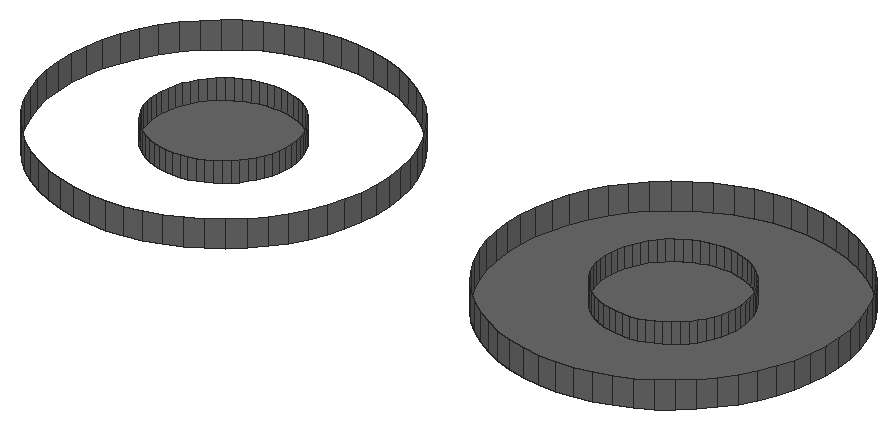
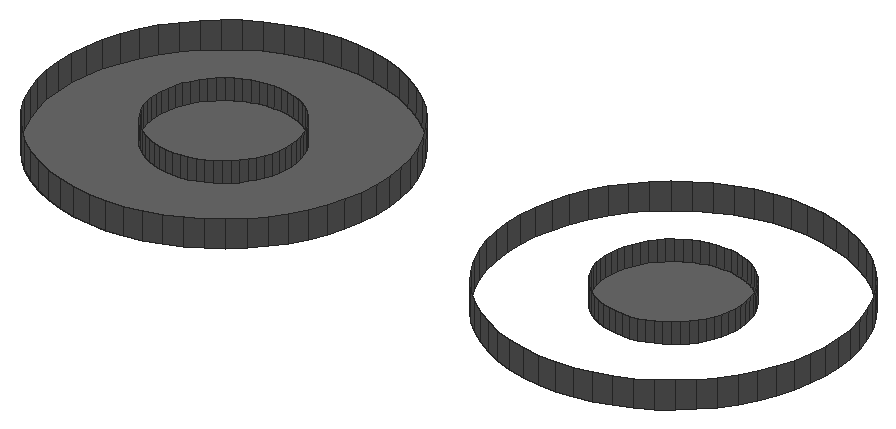
# SketchUp Ruby script. Lengths in inches.
U = 1.inch
M = Sketchup.active_model
def pt(a) = Geom::Point3d.new(a.map { |v| v * U })
def face(e, loops, mat)
  f = e.add_face(loops[0].map { |a| pt(a) })
  loops[1..].each { |l| e.add_face(l.map { |a| pt(a) }).erase! }
  f.material = f.back_material = mat if mat
  f
end
# faces: each face lists its corners as indices into pts; further lists are holes
def faces(e, pts, list, mat = nil) = list.each { |f| face(e, (f[0].is_a?(Array) ? f : [f]).map { |l| l.map { |i| pts[i] } }, mat) }
# xy, xz, yz: faces in a plane at the given z, y or x. An outline is a flat list of corners, or four numbers for a rectangle; further outlines are holes
def ring(l) = l.size == 4 ? [[l[0], l[1]], [l[2], l[1]], [l[2], l[3]], [l[0], l[3]]] : l.each_slice(2).to_a
def flat(e, list, mat, &to3) = list.each { |f| face(e, (f[0].is_a?(Array) ? f : [f]).map { |l| ring(l).map { |u, v| to3.(u, v) } }, mat) }
def xy(e, z, list, mat = nil) = flat(e, list, mat) { |x, y| [x, y, z] }
def xz(e, y, list, mat = nil) = flat(e, list, mat) { |x, z| [x, y, z] }
def yz(e, x, list, mat = nil) = flat(e, list, mat) { |y, z| [x, y, z] }
def lines(e, pts, list) = list.each { |a, b| e.add_line(pt(pts[a]), pt(pts[b])) }
# prism: a flat outline (further loops are holes) pulled along v
def prism(e, loops, v, mat = nil)
  f = face(e, loops, mat); d = Geom::Vector3d.new(v.map { |x| x * U })
  f.pushpull(f.normal.samedirection?(d) ? d.length : -d.length)
end
def box(e, o, s, mat = nil) = prism(e, [[o, [o[0] + s[0], o[1], o[2]], [o[0] + s[0], o[1] + s[1], o[2]], [o[0], o[1] + s[1], o[2]]]], [0, 0, s[2]], mat)
def at(x, y, z, deg = 0) = Geom::Transformation.translation(pt([x, y, z])) * Geom::Transformation.rotation(ORIGIN, Z_AXIS, deg.degrees)
def axes(o, x, y, z) = Geom::Transformation.new([*x, 0, *y, 0, *z, 0, *pt(o).to_a, 1])
def part(name) = M.definitions.add(name)
# library, detail: a bought-in or finely detailed component or shape, given as its bounding box
def library(name, o, s) = part(name).tap { |d| box(d.entities, o, s) }
def detail(e, o, s) = box(e.add_group.entities, o, s)
def put(e, d, t, mat = nil) = e.add_instance(d, t).tap { |i| i.material = mat if mat }
def group(e, t, mat = nil) = e.add_group.tap { |g| g.transformation = t; g.material = mat if mat }.entities
root = M.entities
M.materials.add("[0134_DimGray]").color = [105, 105, 105]
xy(root,118,[[107.89,159.41,106.64,159.53,105.41,159.78,104.21,160.16,103.0625,160.67,101.97,161.29,100.95,162.02,100.01,162.85,99.16,163.78,98.42,164.79,97.78,165.875,97.26,167.02,96.87,168.21,96.6,169.4375,96.46,170.6875,96.45,171.94,96.57,173.19,96.83,174.42,97.21,175.62,97.71,176.77,98.33,177.86,99.0625,178.88,99.9,179.82,100.82,180.67,101.84,181.42,102.92,182.05,104.0625,182.57,105.26,182.97,106.48,183.23,107.73,183.375,108.99,183.38,110.24,183.26,111.47,183.01,112.66,182.625,113.81,182.125,114.91,181.5,115.93,180.77,116.87,179.9375,117.71,179.01,118.46,178,119.09,176.91,119.61,175.77,120.01,174.58,120.28,173.35,120.42,172.1,120.43,170.85,120.3,169.6,120.05,168.37,119.67,167.17,119.17,166.02,118.55,164.93,117.8125,163.91,116.98,162.97,116.05,162.12,115.04,161.375,113.96,160.74,112.8125,160.22,111.62,159.83,110.39,159.56,109.15,159.42]],"[0134_DimGray]")
xy(root,118.5,[[75.77,164.98,76.3,165.02,76.81,165.12,77.31,165.28,77.79,165.48,78.25,165.73,78.68,166.03,79.07,166.38,79.43,166.76,79.75,167.18,80.01,167.625,80.24,168.1,80.41,168.6,80.52,169.11,80.59,169.625,80.6,170.15,80.55,170.67,80.45,171.18,80.3,171.68,80.09,172.17,79.84,172.625,79.54,173.05,79.2,173.45,78.8125,173.8,78.4,174.12,77.95,174.39,77.47,174.61,76.98,174.78,76.47,174.9,75.95,174.96,75.43,174.97,74.9,174.93,74.39,174.83,73.89,174.67,73.41,174.47,72.95,174.21,72.52,173.91,72.125,173.57,71.77,173.1875,71.45,172.77,71.19,172.32,70.96,171.85,70.79,171.35,70.68,170.84,70.61,170.32,70.6,169.8,70.65,169.28,70.75,168.76,70.9,168.26,71.11,167.78,71.36,167.32,71.66,166.9,72,166.5,72.39,166.14,72.8,165.83,73.25,165.56,73.73,165.34,74.22,165.17,74.73,165.05,75.25,164.99],[108.61,166.4,109.13,166.44,109.65,166.54,110.15,166.7,110.63,166.9,111.09,167.16,111.52,167.46,111.91,167.8,112.27,168.18,112.58,168.6,112.85,169.05,113.07,169.52,113.24,170.02,113.36,170.53,113.43,171.05,113.44,171.57,113.39,172.09,113.29,172.6,113.14,173.11,112.93,173.59,112.68,174.04,112.38,174.47,112.03,174.87,111.65,175.23,111.23,175.54,110.79,175.81,110.3125,176.03,109.82,176.2,109.31,176.32,108.79,176.38,108.26,176.39,107.74,176.35,107.23,176.25,106.73,176.09,106.25,175.89,105.79,175.64,105.36,175.34,104.96,174.99,104.61,174.61,104.29,174.19,104.02,173.74,103.8,173.27,103.63,172.77,103.51,172.26,103.45,171.74,103.44,171.22,103.49,170.7,103.59,170.1875,103.74,169.69,103.94,169.2,104.2,168.75,104.5,168.32,104.84,167.92,105.22,167.57,105.64,167.25,106.09,166.98,106.57,166.76,107.06,166.59,107.57,166.47,108.09,166.41]],"[0134_DimGray]")
p = [[73.8,158.11,118],[75.05,157.99,118],[75.05,157.99,120],[73.8,158.11,120],[76.31,158,118],[76.31,158,120],
  [77.56,158.13,118],[77.56,158.13,120],[72.57,158.36,118],[72.57,158.36,120],[78.78,158.4,118],[78.78,158.4,120],
  [71.375,158.74,118],[71.375,158.74,120],[79.98,158.8,118],[79.98,158.8,120],[70.22,159.25,118],[70.22,159.25,120],
  [81.12,159.32,118],[81.12,159.32,120],[69.13,159.87,118],[69.13,159.87,120],[82.2,159.95,118],[82.2,159.95,120],
  [106.64,159.53,118],[107.89,159.41,118],[107.89,159.41,120],[106.64,159.53,120],[109.15,159.42,118],[109.15,159.42,120],
  [110.39,159.56,118],[110.39,159.56,120],[105.41,159.78,118],[105.41,159.78,120],[111.62,159.83,118],[111.62,159.83,120],
  [104.21,160.16,118],[104.21,160.16,120],[112.8125,160.22,118],[112.8125,160.22,120],[68.11,160.6,118],[68.11,160.6,120],
  [83.21,160.7,118],[83.21,160.7,120],[103.0625,160.67,118],[103.0625,160.67,120],[113.96,160.74,118],[113.96,160.74,120],
  [67.17,161.43,118],[67.17,161.43,120],[84.14,161.55,118],[84.14,161.55,120],[101.97,161.29,118],[101.97,161.29,120],
  [115.04,161.375,118],[115.04,161.375,120],[100.95,162.02,118],[100.95,162.02,120],[66.33,162.36,118],[66.33,162.36,120],
  [116.05,162.12,118],[116.05,162.12,120],[84.98,162.48,118],[84.98,162.48,120],[100.01,162.85,118],[100.01,162.85,120],
  [116.98,162.97,118],[116.98,162.97,120],[65.58,163.37,118],[65.58,163.37,120],[85.71,163.51,118],[85.71,163.51,120],
  [99.16,163.78,118],[99.16,163.78,120],[117.8125,163.91,118],[117.8125,163.91,120],[64.94,164.46,118],[64.94,164.46,120],
  [86.33,164.6,118],[86.33,164.6,120],[98.42,164.79,118],[98.42,164.79,120],[118.55,164.93,118],[118.55,164.93,120],
  [64.43,165.6,118],[64.43,165.6,120],[86.83,165.75,118],[86.83,165.75,120],[97.78,165.875,118],[97.78,165.875,120],
  [119.17,166.02,118],[119.17,166.02,120],[64.03,166.79,118],[64.03,166.79,120],[87.21,166.95,118],[87.21,166.95,120],
  [97.26,167.02,118],[97.26,167.02,120],[119.67,167.17,118],[119.67,167.17,120],[63.76,168.02,118],[63.76,168.02,120],
  [87.46,168.18,118],[87.46,168.18,120],[96.87,168.21,118],[96.87,168.21,120],[120.05,168.37,118],[120.05,168.37,120],
  [63.62,169.27,118],[63.62,169.27,120],[87.59,169.43,118],[87.59,169.43,120],[96.6,169.4375,118],[96.6,169.4375,120],
  [120.3,169.6,118],[120.3,169.6,120],[63.61,170.52,118],[63.61,170.52,120],[87.58,170.68,118],[87.58,170.68,120],
  [96.46,170.6875,118],[96.46,170.6875,120],[120.43,170.85,118],[120.43,170.85,120],[63.74,171.77,118],[63.74,171.77,120],
  [87.44,171.93,118],[87.44,171.93,120],[96.45,171.94,118],[96.45,171.94,120],[120.42,172.1,118],[120.42,172.1,120],
  [63.99,173,118],[63.99,173,120],[87.17,173.16,118],[87.17,173.16,120],[96.57,173.19,118],[96.57,173.19,120],
  [120.28,173.35,118],[120.28,173.35,120],[64.37,174.2,118],[64.37,174.2,120],[86.77,174.35,118],[86.77,174.35,120],
  [96.83,174.42,118],[96.83,174.42,120],[120.01,174.58,118],[120.01,174.58,120],[64.87,175.35,118],[64.87,175.35,120],
  [86.26,175.49,118],[86.26,175.49,120],[97.21,175.62,118],[97.21,175.62,120],[119.61,175.77,118],[119.61,175.77,120],
  [65.49,176.44,118],[65.49,176.44,120],[85.62,176.58,118],[85.62,176.58,120],[97.71,176.77,118],[97.71,176.77,120],
  [119.09,176.91,118],[119.09,176.91,120],[66.22,177.46,118],[66.22,177.46,120],[84.875,177.59,118],[84.875,177.59,120],
  [98.33,177.86,118],[98.33,177.86,120],[118.46,178,118],[118.46,178,120],[67.06,178.4,118],[67.06,178.4,120],
  [84.03,178.52,118],[84.03,178.52,120],[99.0625,178.88,118],[99.0625,178.88,120],[117.71,179.01,118],[117.71,179.01,120],
  [67.99,179.25,118],[67.99,179.25,120],[83.09,179.35,118],[83.09,179.35,120],[99.9,179.82,118],[99.9,179.82,120],
  [116.87,179.9375,118],[116.87,179.9375,120],[69,179.99,118],[69,179.99,120],[82.07,180.08,118],[82.07,180.08,120],
  [100.82,180.67,118],[100.82,180.67,120],[115.93,180.77,118],[115.93,180.77,120],[70.08,180.63,118],[70.08,180.63,120],
  [80.98,180.7,118],[80.98,180.7,120],[71.23,181.15,118],[71.23,181.15,120],[79.83,181.21,118],[79.83,181.21,120],
  [101.84,181.42,118],[101.84,181.42,120],[114.91,181.5,118],[114.91,181.5,120],[72.42,181.54,118],[72.42,181.54,120],
  [78.63,181.59,118],[78.63,181.59,120],[102.92,182.05,118],[102.92,182.05,120],[73.64,181.8125,118],[73.64,181.8125,120],
  [113.81,182.125,118],[113.81,182.125,120],[77.4,181.84,118],[77.4,181.84,120],[74.89,181.95,118],[74.89,181.95,120],
  [76.15,181.96,118],[76.15,181.96,120],[104.0625,182.57,118],[104.0625,182.57,120],[112.66,182.625,118],[112.66,182.625,120],
  [105.26,182.97,118],[105.26,182.97,120],[111.47,183.01,118],[111.47,183.01,120],[106.48,183.23,118],[106.48,183.23,120],
  [110.24,183.26,118],[110.24,183.26,120],[107.73,183.375,118],[107.73,183.375,120],[108.99,183.38,118],[108.99,183.38,120],
  [74.73,165.05,120],[75.25,164.99,120],[75.25,164.99,118.5],[74.73,165.05,118.5],[75.77,164.98,120],[75.77,164.98,118.5],
  [76.3,165.02,120],[76.3,165.02,118.5],[76.81,165.12,120],[76.81,165.12,118.5],[74.22,165.17,120],[74.22,165.17,118.5],
  [77.31,165.28,120],[77.31,165.28,118.5],[73.73,165.34,120],[73.73,165.34,118.5],[73.25,165.56,120],[73.25,165.56,118.5],
  [77.79,165.48,120],[77.79,165.48,118.5],[78.25,165.73,120],[78.25,165.73,118.5],[72.8,165.83,120],[72.8,165.83,118.5],
  [78.68,166.03,120],[78.68,166.03,118.5],[72.39,166.14,120],[72.39,166.14,118.5],[79.07,166.38,120],[79.07,166.38,118.5],
  [72,166.5,120],[72,166.5,118.5],[79.43,166.76,120],[79.43,166.76,118.5],[107.57,166.47,120],[108.09,166.41,120],
  [108.09,166.41,118.5],[107.57,166.47,118.5],[108.61,166.4,120],[108.61,166.4,118.5],[109.13,166.44,120],[109.13,166.44,118.5],
  [109.65,166.54,120],[109.65,166.54,118.5],[71.66,166.9,120],[71.66,166.9,118.5],[107.06,166.59,120],[107.06,166.59,118.5],
  [110.15,166.7,120],[110.15,166.7,118.5],[106.57,166.76,120],[106.57,166.76,118.5],[110.63,166.9,120],[110.63,166.9,118.5],
  [79.75,167.18,120],[79.75,167.18,118.5],[106.09,166.98,120],[106.09,166.98,118.5],[71.36,167.32,120],[71.36,167.32,118.5],
  [111.09,167.16,120],[111.09,167.16,118.5],[105.64,167.25,120],[105.64,167.25,118.5],[80.01,167.625,120],[80.01,167.625,118.5],
  [111.52,167.46,120],[111.52,167.46,118.5],[71.11,167.78,120],[71.11,167.78,118.5],[105.22,167.57,120],[105.22,167.57,118.5],
  [111.91,167.8,120],[111.91,167.8,118.5],[80.24,168.1,120],[80.24,168.1,118.5],[104.84,167.92,120],[104.84,167.92,118.5],
  [70.9,168.26,120],[70.9,168.26,118.5],[112.27,168.18,120],[112.27,168.18,118.5],[104.5,168.32,120],[104.5,168.32,118.5],
  [80.41,168.6,120],[80.41,168.6,118.5],[112.58,168.6,120],[112.58,168.6,118.5],[70.75,168.76,120],[70.75,168.76,118.5],
  [104.2,168.75,120],[104.2,168.75,118.5],[80.52,169.11,120],[80.52,169.11,118.5],[112.85,169.05,120],[112.85,169.05,118.5],
  [103.94,169.2,120],[103.94,169.2,118.5],[70.65,169.28,120],[70.65,169.28,118.5],[113.07,169.52,120],[113.07,169.52,118.5],
  [80.59,169.625,120],[80.59,169.625,118.5],[103.74,169.69,120],[103.74,169.69,118.5],[70.6,169.8,120],[70.6,169.8,118.5],
  [113.24,170.02,120],[113.24,170.02,118.5],[80.6,170.15,120],[80.6,170.15,118.5],[103.59,170.1875,120],[103.59,170.1875,118.5],
  [70.61,170.32,120],[70.61,170.32,118.5],[113.36,170.53,120],[113.36,170.53,118.5],[80.55,170.67,120],[80.55,170.67,118.5],
  [103.49,170.7,120],[103.49,170.7,118.5],[70.68,170.84,120],[70.68,170.84,118.5],[113.43,171.05,120],[113.43,171.05,118.5],
  [80.45,171.18,120],[80.45,171.18,118.5],[103.44,171.22,120],[103.44,171.22,118.5],[70.79,171.35,120],[70.79,171.35,118.5],
  [113.44,171.57,120],[113.44,171.57,118.5],[80.3,171.68,120],[80.3,171.68,118.5],[103.45,171.74,120],[103.45,171.74,118.5],
  [70.96,171.85,120],[70.96,171.85,118.5],[113.39,172.09,120],[113.39,172.09,118.5],[80.09,172.17,120],[80.09,172.17,118.5],
  [103.51,172.26,120],[103.51,172.26,118.5],[71.19,172.32,120],[71.19,172.32,118.5],[113.29,172.6,120],[113.29,172.6,118.5],
  [79.84,172.625,120],[79.84,172.625,118.5],[71.45,172.77,120],[71.45,172.77,118.5],[103.63,172.77,120],[103.63,172.77,118.5],
  [79.54,173.05,120],[79.54,173.05,118.5],[113.14,173.11,120],[113.14,173.11,118.5],[71.77,173.1875,120],[71.77,173.1875,118.5],
  [103.8,173.27,120],[103.8,173.27,118.5],[79.2,173.45,120],[79.2,173.45,118.5],[112.93,173.59,120],[112.93,173.59,118.5],
  [72.125,173.57,120],[72.125,173.57,118.5],[104.02,173.74,120],[104.02,173.74,118.5],[78.8125,173.8,120],[78.8125,173.8,118.5],
  [72.52,173.91,120],[72.52,173.91,118.5],[112.68,174.04,120],[112.68,174.04,118.5],[104.29,174.19,120],[104.29,174.19,118.5],
  [78.4,174.12,120],[78.4,174.12,118.5],[72.95,174.21,120],[72.95,174.21,118.5],[112.38,174.47,120],[112.38,174.47,118.5],
  [77.95,174.39,120],[77.95,174.39,118.5],[73.41,174.47,120],[73.41,174.47,118.5],[104.61,174.61,120],[104.61,174.61,118.5],
  [77.47,174.61,120],[77.47,174.61,118.5],[73.89,174.67,120],[73.89,174.67,118.5],[112.03,174.87,120],[112.03,174.87,118.5],
  [76.98,174.78,120],[76.98,174.78,118.5],[104.96,174.99,120],[104.96,174.99,118.5],[74.39,174.83,120],[74.39,174.83,118.5],
  [74.9,174.93,120],[74.9,174.93,118.5],[76.47,174.9,120],[76.47,174.9,118.5],[75.43,174.97,120],[75.43,174.97,118.5],
  [75.95,174.96,120],[75.95,174.96,118.5],[111.65,175.23,120],[111.65,175.23,118.5],[105.36,175.34,120],[105.36,175.34,118.5],
  [111.23,175.54,120],[111.23,175.54,118.5],[105.79,175.64,120],[105.79,175.64,118.5],[110.79,175.81,120],[110.79,175.81,118.5],
  [106.25,175.89,120],[106.25,175.89,118.5],[110.3125,176.03,120],[110.3125,176.03,118.5],[106.73,176.09,120],[106.73,176.09,118.5],
  [109.82,176.2,120],[109.82,176.2,118.5],[107.23,176.25,120],[107.23,176.25,118.5],[107.74,176.35,120],[107.74,176.35,118.5],
  [109.31,176.32,120],[109.31,176.32,118.5],[108.26,176.39,120],[108.26,176.39,118.5],[108.79,176.38,120],[108.79,176.38,118.5]]
faces(root,p,[[0,1,2,3],[1,4,5,2],[4,6,7,5],[8,0,3,9],[6,10,11,7],[12,8,9,13],[10,14,15,11],[16,12,13,17],
  [14,18,19,15],[20,16,17,21],[18,22,23,19],[24,25,26,27],[25,28,29,26],[28,30,31,29],[32,24,27,33],[30,34,35,31],
  [36,32,33,37],[34,38,39,35],[40,20,21,41],[22,42,43,23],[44,36,37,45],[38,46,47,39],[48,40,41,49],[42,50,51,43],
  [52,44,45,53],[46,54,55,47],[56,52,53,57],[58,48,49,59],[54,60,61,55],[50,62,63,51],[64,56,57,65],[60,66,67,61],
  [68,58,59,69],[62,70,71,63],[72,64,65,73],[66,74,75,67],[76,68,69,77],[70,78,79,71],[80,72,73,81],[74,82,83,75],
  [84,76,77,85],[78,86,87,79],[88,80,81,89],[82,90,91,83],[92,84,85,93],[86,94,95,87],[96,88,89,97],[90,98,99,91],
  [100,92,93,101],[94,102,103,95],[104,96,97,105],[98,106,107,99],[108,100,101,109],[102,110,111,103],[112,104,105,113],[106,114,115,107],
  [116,108,109,117],[110,118,119,111],[120,112,113,121],[114,122,123,115],[124,116,117,125],[118,126,127,119],[128,120,121,129],[122,130,131,123],
  [132,124,125,133],[126,134,135,127],[136,128,129,137],[130,138,139,131],[140,132,133,141],[134,142,143,135],[144,136,137,145],[138,146,147,139],
  [148,140,141,149],[142,150,151,143],[152,144,145,153],[146,154,155,147],[156,148,149,157],[150,158,159,151],[160,152,153,161],[154,162,163,155],
  [164,156,157,165],[158,166,167,159],[168,160,161,169],[162,170,171,163],[172,164,165,173],[166,174,175,167],[176,168,169,177],[170,178,179,171],
  [180,172,173,181],[174,182,183,175],[184,176,177,185],[178,186,187,179],[188,180,181,189],[182,190,191,183],[192,184,185,193],[186,194,195,187],
  [196,188,189,197],[190,198,199,191],[200,196,197,201],[198,202,203,199],[204,192,193,205],[194,206,207,195],[208,200,201,209],[202,210,211,203],
  [212,204,205,213],[214,208,209,215],[206,216,217,207],[210,218,219,211],[220,214,215,221],[218,222,223,219],[222,220,221,223],[224,212,213,225],
  [216,226,227,217],[228,224,225,229],[226,230,231,227],[232,228,229,233],[230,234,235,231],[236,232,233,237],[234,238,239,235],[238,236,237,239],
  [240,241,242,243],[241,244,245,242],[244,246,247,245],[246,248,249,247],[250,240,243,251],[248,252,253,249],[254,250,251,255],[256,254,255,257],
  [252,258,259,253],[258,260,261,259],[262,256,257,263],[260,264,265,261],[266,262,263,267],[264,268,269,265],[270,266,267,271],[268,272,273,269],
  [274,275,276,277],[275,278,279,276],[278,280,281,279],[280,282,283,281],[284,270,271,285],[286,274,277,287],[282,288,289,283],[290,286,287,291],
  [288,292,293,289],[272,294,295,273],[296,290,291,297],[298,284,285,299],[292,300,301,293],[302,296,297,303],[294,304,305,295],[300,306,307,301],
  [308,298,299,309],[310,302,303,311],[306,312,313,307],[304,314,315,305],[316,310,311,317],[318,308,309,319],[312,320,321,313],[322,316,317,323],
  [314,324,325,315],[320,326,327,321],[328,318,319,329],[330,322,323,331],[324,332,333,325],[326,334,335,327],[336,330,331,337],[338,328,329,339],
  [334,340,341,335],[332,342,343,333],[344,336,337,345],[346,338,339,347],[340,348,349,341],[342,350,351,343],[352,344,345,353],[354,346,347,355],
  [348,356,357,349],[350,358,359,351],[360,352,353,361],[362,354,355,363],[356,364,365,357],[358,366,367,359],[368,360,361,369],[370,362,363,371],
  [364,372,373,365],[366,374,375,367],[376,368,369,377],[378,370,371,379],[372,380,381,373],[374,382,383,375],[384,376,377,385],[386,378,379,387],
  [380,388,389,381],[382,390,391,383],[392,386,387,393],[394,384,385,395],[390,396,397,391],[388,398,399,389],[400,392,393,401],[402,394,395,403],
  [396,404,405,397],[398,406,407,399],[408,400,401,409],[410,402,403,411],[404,412,413,405],[414,408,409,415],[406,416,417,407],[418,410,411,419],
  [412,420,421,413],[422,414,415,423],[416,424,425,417],[420,426,427,421],[428,422,423,429],[430,418,419,431],[426,432,433,427],[434,428,429,435],
  [424,436,437,425],[432,438,439,433],[440,430,431,441],[442,434,435,443],[444,442,443,445],[438,446,447,439],[448,444,445,449],[446,450,451,447],
  [436,452,453,437],[450,448,449,451],[454,440,441,455],[452,456,457,453],[458,454,455,459],[456,460,461,457],[462,458,459,463],[460,464,465,461],
  [466,462,463,467],[464,468,469,465],[470,466,467,471],[472,470,471,473],[468,474,475,469],[476,472,473,477],[474,478,479,475],[478,476,477,479]],"[0134_DimGray]")
